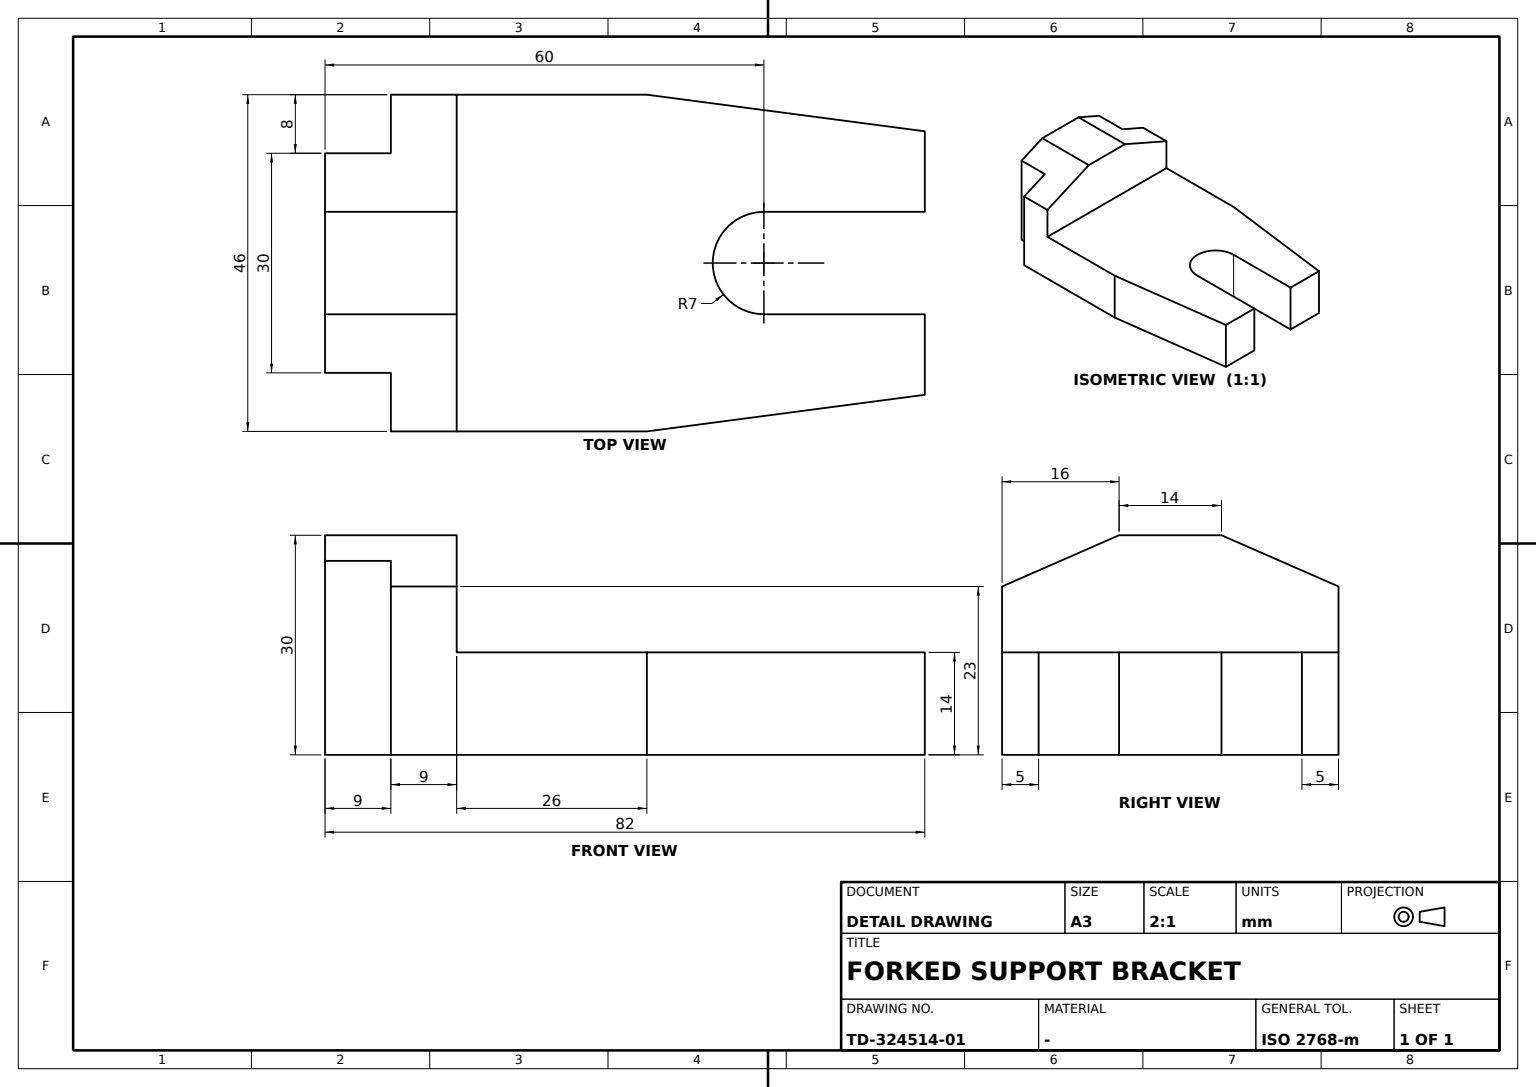
ISO-10303-21;
HEADER;
FILE_DESCRIPTION((''),'2;1');
FILE_NAME('','',(''),(''),'','','');
FILE_SCHEMA(('AUTOMOTIVE_DESIGN'));
ENDSEC;
DATA;
#1=APPLICATION_CONTEXT('');
#2=PRODUCT_CONTEXT('',#1,'mechanical');
#3=PRODUCT('','','',(#2));
#4=PRODUCT_DEFINITION_FORMATION('','',#3);
#5=PRODUCT_DEFINITION_CONTEXT('',#1,'design');
#6=PRODUCT_DEFINITION('','',#4,#5);
#7=PRODUCT_DEFINITION_SHAPE('','',#6);
#8=(LENGTH_UNIT()NAMED_UNIT(*)SI_UNIT(.MILLI.,.METRE.));
#9=(NAMED_UNIT(*)PLANE_ANGLE_UNIT()SI_UNIT($,.RADIAN.));
#10=(NAMED_UNIT(*)SI_UNIT($,.STERADIAN.)SOLID_ANGLE_UNIT());
#11=UNCERTAINTY_MEASURE_WITH_UNIT(LENGTH_MEASURE(0.005),#8,'distance_accuracy_value','');
#12=(GEOMETRIC_REPRESENTATION_CONTEXT(3)GLOBAL_UNCERTAINTY_ASSIGNED_CONTEXT((#11))GLOBAL_UNIT_ASSIGNED_CONTEXT((#8,#9,#10))REPRESENTATION_CONTEXT('',''));
#13=CARTESIAN_POINT('',(60.,-7.,14.));
#14=VERTEX_POINT('',#13);
#15=CARTESIAN_POINT('',(60.,-7.,0.));
#16=VERTEX_POINT('',#15);
#17=CARTESIAN_POINT('',(60.,-7.,-32.));
#18=DIRECTION('',(0.,0.,-1.));
#19=VECTOR('',#18,1000.);
#20=LINE('',#17,#19);
#21=EDGE_CURVE('',#14,#16,#20,.T.);
#22=ORIENTED_EDGE('',*,*,#21,.F.);
#23=CARTESIAN_POINT('',(82.,-7.,14.));
#24=VERTEX_POINT('',#23);
#25=DIRECTION('',(1.,0.,0.));
#26=VECTOR('',#25,1000.);
#27=LINE('',#13,#26);
#28=EDGE_CURVE('',#14,#24,#27,.T.);
#29=ORIENTED_EDGE('',*,*,#28,.T.);
#30=CARTESIAN_POINT('',(82.,-7.,0.));
#31=VERTEX_POINT('',#30);
#32=CARTESIAN_POINT('',(82.,-7.,-32.));
#33=DIRECTION('',(0.,0.,1.));
#34=VECTOR('',#33,1000.);
#35=LINE('',#32,#34);
#36=EDGE_CURVE('',#31,#24,#35,.T.);
#37=ORIENTED_EDGE('',*,*,#36,.F.);
#38=CARTESIAN_POINT('',(0.,-7.,0.));
#39=LINE('',#38,#26);
#40=EDGE_CURVE('',#16,#31,#39,.T.);
#41=ORIENTED_EDGE('',*,*,#40,.F.);
#42=EDGE_LOOP('',(#22,#29,#37,#41));
#43=FACE_BOUND('',#42,.T.);
#44=DIRECTION('',(0.,-1.,0.));
#45=AXIS2_PLACEMENT_3D('',#17,#44,#25);
#46=PLANE('',#45);
#47=ADVANCED_FACE('',(#43),#46,.F.);
#48=CARTESIAN_POINT('',(0.,-15.,0.));
#49=VERTEX_POINT('',#48);
#50=CARTESIAN_POINT('',(0.,-15.,26.5));
#51=VERTEX_POINT('',#50);
#52=CARTESIAN_POINT('',(0.,-15.,-16.));
#53=LINE('',#52,#34);
#54=EDGE_CURVE('',#49,#51,#53,.T.);
#55=ORIENTED_EDGE('',*,*,#54,.F.);
#56=CARTESIAN_POINT('',(9.,-15.,0.));
#57=VERTEX_POINT('',#56);
#58=DIRECTION('',(-1.,0.,0.));
#59=VECTOR('',#58,1000.);
#60=LINE('',#48,#59);
#61=EDGE_CURVE('',#57,#49,#60,.T.);
#62=ORIENTED_EDGE('',*,*,#61,.F.);
#63=CARTESIAN_POINT('',(9.,-15.,26.5));
#64=VERTEX_POINT('',#63);
#65=CARTESIAN_POINT('',(9.,-15.,-16.));
#66=LINE('',#65,#19);
#67=EDGE_CURVE('',#64,#57,#66,.T.);
#68=ORIENTED_EDGE('',*,*,#67,.F.);
#69=LINE('',#63,#59);
#70=EDGE_CURVE('',#64,#51,#69,.T.);
#71=ORIENTED_EDGE('',*,*,#70,.T.);
#72=EDGE_LOOP('',(#55,#62,#68,#71));
#73=FACE_BOUND('',#72,.T.);
#74=DIRECTION('',(0.,1.,0.));
#75=AXIS2_PLACEMENT_3D('',#65,#74,#33);
#76=PLANE('',#75);
#77=ADVANCED_FACE('',(#73),#76,.F.);
#78=CARTESIAN_POINT('',(44.,-23.,0.));
#79=VERTEX_POINT('',#78);
#80=CARTESIAN_POINT('',(44.,-23.,14.));
#81=VERTEX_POINT('',#80);
#82=CARTESIAN_POINT('',(44.,-23.,-32.));
#83=LINE('',#82,#34);
#84=EDGE_CURVE('',#79,#81,#83,.T.);
#85=ORIENTED_EDGE('',*,*,#84,.T.);
#86=CARTESIAN_POINT('',(18.,-23.,14.));
#87=VERTEX_POINT('',#86);
#88=CARTESIAN_POINT('',(82.,-23.,14.));
#89=LINE('',#88,#59);
#90=EDGE_CURVE('',#81,#87,#89,.T.);
#91=ORIENTED_EDGE('',*,*,#90,.T.);
#92=CARTESIAN_POINT('',(18.,-23.,23.));
#93=VERTEX_POINT('',#92);
#94=LINE('',#86,#34);
#95=EDGE_CURVE('',#87,#93,#94,.T.);
#96=ORIENTED_EDGE('',*,*,#95,.T.);
#97=CARTESIAN_POINT('',(9.,-23.,23.));
#98=VERTEX_POINT('',#97);
#99=CARTESIAN_POINT('',(-28.,-23.,23.));
#100=LINE('',#99,#26);
#101=EDGE_CURVE('',#98,#93,#100,.T.);
#102=ORIENTED_EDGE('',*,*,#101,.F.);
#103=CARTESIAN_POINT('',(9.,-23.,0.));
#104=VERTEX_POINT('',#103);
#105=CARTESIAN_POINT('',(9.,-23.,-16.));
#106=LINE('',#105,#34);
#107=EDGE_CURVE('',#104,#98,#106,.T.);
#108=ORIENTED_EDGE('',*,*,#107,.F.);
#109=CARTESIAN_POINT('',(0.,-23.,0.));
#110=LINE('',#109,#26);
#111=EDGE_CURVE('',#104,#79,#110,.T.);
#112=ORIENTED_EDGE('',*,*,#111,.T.);
#113=EDGE_LOOP('',(#85,#91,#96,#102,#108,#112));
#114=FACE_BOUND('',#113,.T.);
#115=AXIS2_PLACEMENT_3D('',#109,#44,#18);
#116=PLANE('',#115);
#117=ADVANCED_FACE('',(#114),#116,.T.);
#118=ORIENTED_EDGE('',*,*,#54,.T.);
#119=CARTESIAN_POINT('',(0.,-7.,30.));
#120=VERTEX_POINT('',#119);
#121=CARTESIAN_POINT('',(0.,-20.429508,24.12459));
#122=DIRECTION('',(0.,0.916157335,0.400818834));
#123=VECTOR('',#122,1000.);
#124=LINE('',#121,#123);
#125=EDGE_CURVE('',#51,#120,#124,.T.);
#126=ORIENTED_EDGE('',*,*,#125,.T.);
#127=CARTESIAN_POINT('',(0.,7.,30.));
#128=VERTEX_POINT('',#127);
#129=CARTESIAN_POINT('',(0.,-23.,30.));
#130=VECTOR('',#74,1000.);
#131=LINE('',#129,#130);
#132=EDGE_CURVE('',#120,#128,#131,.T.);
#133=ORIENTED_EDGE('',*,*,#132,.T.);
#134=CARTESIAN_POINT('',(0.,15.,26.5));
#135=VERTEX_POINT('',#134);
#136=CARTESIAN_POINT('',(0.,-18.180328,41.016393));
#137=DIRECTION('',(0.,0.916157335,-0.400818834));
#138=VECTOR('',#137,1000.);
#139=LINE('',#136,#138);
#140=EDGE_CURVE('',#128,#135,#139,.T.);
#141=ORIENTED_EDGE('',*,*,#140,.T.);
#142=CARTESIAN_POINT('',(0.,15.,0.));
#143=VERTEX_POINT('',#142);
#144=CARTESIAN_POINT('',(0.,15.,-16.));
#145=LINE('',#144,#34);
#146=EDGE_CURVE('',#143,#135,#145,.T.);
#147=ORIENTED_EDGE('',*,*,#146,.F.);
#148=LINE('',#109,#130);
#149=EDGE_CURVE('',#49,#143,#148,.T.);
#150=ORIENTED_EDGE('',*,*,#149,.F.);
#151=EDGE_LOOP('',(#118,#126,#133,#141,#147,#150));
#152=FACE_BOUND('',#151,.T.);
#153=AXIS2_PLACEMENT_3D('',#129,#25,#18);
#154=PLANE('',#153);
#155=ADVANCED_FACE('',(#152),#154,.F.);
#156=CARTESIAN_POINT('',(18.,23.,14.));
#157=VERTEX_POINT('',#156);
#158=CARTESIAN_POINT('',(18.,23.,23.));
#159=VERTEX_POINT('',#158);
#160=LINE('',#156,#34);
#161=EDGE_CURVE('',#157,#159,#160,.T.);
#162=ORIENTED_EDGE('',*,*,#161,.F.);
#163=CARTESIAN_POINT('',(44.,23.,14.));
#164=VERTEX_POINT('',#163);
#165=CARTESIAN_POINT('',(82.,23.,14.));
#166=LINE('',#165,#59);
#167=EDGE_CURVE('',#164,#157,#166,.T.);
#168=ORIENTED_EDGE('',*,*,#167,.F.);
#169=CARTESIAN_POINT('',(44.,23.,0.));
#170=VERTEX_POINT('',#169);
#171=CARTESIAN_POINT('',(44.,23.,-32.));
#172=LINE('',#171,#34);
#173=EDGE_CURVE('',#170,#164,#172,.T.);
#174=ORIENTED_EDGE('',*,*,#173,.F.);
#175=CARTESIAN_POINT('',(9.,23.,0.));
#176=VERTEX_POINT('',#175);
#177=CARTESIAN_POINT('',(0.,23.,0.));
#178=LINE('',#177,#26);
#179=EDGE_CURVE('',#176,#170,#178,.T.);
#180=ORIENTED_EDGE('',*,*,#179,.F.);
#181=CARTESIAN_POINT('',(9.,23.,23.));
#182=VERTEX_POINT('',#181);
#183=CARTESIAN_POINT('',(9.,23.,-16.));
#184=LINE('',#183,#34);
#185=EDGE_CURVE('',#176,#182,#184,.T.);
#186=ORIENTED_EDGE('',*,*,#185,.T.);
#187=CARTESIAN_POINT('',(-28.,23.,23.));
#188=LINE('',#187,#26);
#189=EDGE_CURVE('',#182,#159,#188,.T.);
#190=ORIENTED_EDGE('',*,*,#189,.T.);
#191=EDGE_LOOP('',(#162,#168,#174,#180,#186,#190));
#192=FACE_BOUND('',#191,.T.);
#193=AXIS2_PLACEMENT_3D('',#177,#44,#18);
#194=PLANE('',#193);
#195=ADVANCED_FACE('',(#192),#194,.F.);
#196=CARTESIAN_POINT('',(18.,7.,30.));
#197=VERTEX_POINT('',#196);
#198=LINE('',#196,#138);
#199=EDGE_CURVE('',#197,#159,#198,.T.);
#200=ORIENTED_EDGE('',*,*,#199,.T.);
#201=ORIENTED_EDGE('',*,*,#189,.F.);
#202=CARTESIAN_POINT('',(9.,15.,26.5));
#203=VERTEX_POINT('',#202);
#204=CARTESIAN_POINT('',(9.,30.606557,19.672131));
#205=LINE('',#204,#138);
#206=EDGE_CURVE('',#203,#182,#205,.T.);
#207=ORIENTED_EDGE('',*,*,#206,.F.);
#208=LINE('',#134,#26);
#209=EDGE_CURVE('',#135,#203,#208,.T.);
#210=ORIENTED_EDGE('',*,*,#209,.F.);
#211=ORIENTED_EDGE('',*,*,#140,.F.);
#212=CARTESIAN_POINT('',(-28.,7.,30.));
#213=LINE('',#212,#26);
#214=EDGE_CURVE('',#128,#197,#213,.T.);
#215=ORIENTED_EDGE('',*,*,#214,.T.);
#216=EDGE_LOOP('',(#200,#201,#207,#210,#211,#215));
#217=FACE_BOUND('',#216,.T.);
#218=DIRECTION('',(0.,-0.400818834,-0.916157335));
#219=AXIS2_PLACEMENT_3D('',#212,#218,#137);
#220=PLANE('',#219);
#221=ADVANCED_FACE('',(#217),#220,.F.);
#222=ORIENTED_EDGE('',*,*,#161,.T.);
#223=ORIENTED_EDGE('',*,*,#199,.F.);
#224=CARTESIAN_POINT('',(18.,-7.,30.));
#225=VERTEX_POINT('',#224);
#226=CARTESIAN_POINT('',(18.,-23.,30.));
#227=LINE('',#226,#130);
#228=EDGE_CURVE('',#225,#197,#227,.T.);
#229=ORIENTED_EDGE('',*,*,#228,.F.);
#230=LINE('',#92,#123);
#231=EDGE_CURVE('',#93,#225,#230,.T.);
#232=ORIENTED_EDGE('',*,*,#231,.F.);
#233=ORIENTED_EDGE('',*,*,#95,.F.);
#234=LINE('',#86,#130);
#235=EDGE_CURVE('',#87,#157,#234,.T.);
#236=ORIENTED_EDGE('',*,*,#235,.T.);
#237=EDGE_LOOP('',(#222,#223,#229,#232,#233,#236));
#238=FACE_BOUND('',#237,.T.);
#239=AXIS2_PLACEMENT_3D('',#86,#58,#33);
#240=PLANE('',#239);
#241=ADVANCED_FACE('',(#238),#240,.F.);
#242=ORIENTED_EDGE('',*,*,#21,.T.);
#243=CARTESIAN_POINT('',(60.,7.,0.));
#244=VERTEX_POINT('',#243);
#245=CARTESIAN_POINT('',(60.,0.,0.));
#246=AXIS2_PLACEMENT_3D('',#245,#33,#25);
#247=CIRCLE('',#246,7.);
#248=EDGE_CURVE('',#244,#16,#247,.T.);
#249=ORIENTED_EDGE('',*,*,#248,.F.);
#250=CARTESIAN_POINT('',(60.,7.,14.));
#251=VERTEX_POINT('',#250);
#252=CARTESIAN_POINT('',(60.,7.,-32.));
#253=LINE('',#252,#19);
#254=EDGE_CURVE('',#251,#244,#253,.T.);
#255=ORIENTED_EDGE('',*,*,#254,.F.);
#256=CARTESIAN_POINT('',(60.,0.,14.));
#257=AXIS2_PLACEMENT_3D('',#256,#33,#74);
#258=CIRCLE('',#257,7.);
#259=EDGE_CURVE('',#251,#14,#258,.T.);
#260=ORIENTED_EDGE('',*,*,#259,.T.);
#261=EDGE_LOOP('',(#242,#249,#255,#260));
#262=FACE_BOUND('',#261,.T.);
#263=CARTESIAN_POINT('',(60.,0.,-32.));
#264=AXIS2_PLACEMENT_3D('',#263,#33,#25);
#265=CYLINDRICAL_SURFACE('',#264,7.);
#266=ADVANCED_FACE('',(#262),#265,.F.);
#267=LINE('',#103,#130);
#268=EDGE_CURVE('',#104,#57,#267,.T.);
#269=ORIENTED_EDGE('',*,*,#268,.F.);
#270=ORIENTED_EDGE('',*,*,#107,.T.);
#271=CARTESIAN_POINT('',(9.,-37.321311,16.734426));
#272=LINE('',#271,#123);
#273=EDGE_CURVE('',#98,#64,#272,.T.);
#274=ORIENTED_EDGE('',*,*,#273,.T.);
#275=ORIENTED_EDGE('',*,*,#67,.T.);
#276=EDGE_LOOP('',(#269,#270,#274,#275));
#277=FACE_BOUND('',#276,.T.);
#278=AXIS2_PLACEMENT_3D('',#105,#25,#18);
#279=PLANE('',#278);
#280=ADVANCED_FACE('',(#277),#279,.F.);
#281=CARTESIAN_POINT('',(9.,15.,0.));
#282=VERTEX_POINT('',#281);
#283=CARTESIAN_POINT('',(9.,15.,-16.));
#284=LINE('',#283,#19);
#285=EDGE_CURVE('',#203,#282,#284,.T.);
#286=ORIENTED_EDGE('',*,*,#285,.T.);
#287=LINE('',#142,#26);
#288=EDGE_CURVE('',#143,#282,#287,.T.);
#289=ORIENTED_EDGE('',*,*,#288,.F.);
#290=ORIENTED_EDGE('',*,*,#146,.T.);
#291=ORIENTED_EDGE('',*,*,#209,.T.);
#292=EDGE_LOOP('',(#286,#289,#290,#291));
#293=FACE_BOUND('',#292,.T.);
#294=AXIS2_PLACEMENT_3D('',#144,#44,#18);
#295=PLANE('',#294);
#296=ADVANCED_FACE('',(#293),#295,.F.);
#297=CARTESIAN_POINT('',(82.,7.,14.));
#298=VERTEX_POINT('',#297);
#299=LINE('',#297,#59);
#300=EDGE_CURVE('',#298,#251,#299,.T.);
#301=ORIENTED_EDGE('',*,*,#300,.T.);
#302=ORIENTED_EDGE('',*,*,#254,.T.);
#303=CARTESIAN_POINT('',(82.,7.,0.));
#304=VERTEX_POINT('',#303);
#305=CARTESIAN_POINT('',(0.,7.,0.));
#306=LINE('',#305,#59);
#307=EDGE_CURVE('',#304,#244,#306,.T.);
#308=ORIENTED_EDGE('',*,*,#307,.F.);
#309=CARTESIAN_POINT('',(82.,7.,-32.));
#310=LINE('',#309,#34);
#311=EDGE_CURVE('',#304,#298,#310,.T.);
#312=ORIENTED_EDGE('',*,*,#311,.T.);
#313=EDGE_LOOP('',(#301,#302,#308,#312));
#314=FACE_BOUND('',#313,.T.);
#315=AXIS2_PLACEMENT_3D('',#309,#74,#58);
#316=PLANE('',#315);
#317=ADVANCED_FACE('',(#314),#316,.F.);
#318=CARTESIAN_POINT('',(82.,-18.,0.));
#319=VERTEX_POINT('',#318);
#320=CARTESIAN_POINT('',(0.748809,-28.690946,0.));
#321=DIRECTION('',(-0.991454296,-0.130454513,0.));
#322=VECTOR('',#321,1000.);
#323=LINE('',#320,#322);
#324=EDGE_CURVE('',#319,#79,#323,.T.);
#325=ORIENTED_EDGE('',*,*,#324,.F.);
#326=CARTESIAN_POINT('',(82.,-18.,14.));
#327=VERTEX_POINT('',#326);
#328=CARTESIAN_POINT('',(82.,-18.,-32.));
#329=LINE('',#328,#34);
#330=EDGE_CURVE('',#319,#327,#329,.T.);
#331=ORIENTED_EDGE('',*,*,#330,.T.);
#332=LINE('',#326,#322);
#333=EDGE_CURVE('',#327,#81,#332,.T.);
#334=ORIENTED_EDGE('',*,*,#333,.T.);
#335=ORIENTED_EDGE('',*,*,#84,.F.);
#336=EDGE_LOOP('',(#325,#331,#334,#335));
#337=FACE_BOUND('',#336,.T.);
#338=DIRECTION('',(-0.130454513,0.991454296,0.));
#339=AXIS2_PLACEMENT_3D('',#328,#338,#321);
#340=PLANE('',#339);
#341=ADVANCED_FACE('',(#337),#340,.F.);
#342=ORIENTED_EDGE('',*,*,#167,.T.);
#343=ORIENTED_EDGE('',*,*,#235,.F.);
#344=ORIENTED_EDGE('',*,*,#90,.F.);
#345=ORIENTED_EDGE('',*,*,#333,.F.);
#346=LINE('',#88,#130);
#347=EDGE_CURVE('',#327,#24,#346,.T.);
#348=ORIENTED_EDGE('',*,*,#347,.T.);
#349=ORIENTED_EDGE('',*,*,#28,.F.);
#350=ORIENTED_EDGE('',*,*,#259,.F.);
#351=ORIENTED_EDGE('',*,*,#300,.F.);
#352=CARTESIAN_POINT('',(82.,18.,14.));
#353=VERTEX_POINT('',#352);
#354=EDGE_CURVE('',#298,#353,#346,.T.);
#355=ORIENTED_EDGE('',*,*,#354,.T.);
#356=DIRECTION('',(0.991454296,-0.130454513,0.));
#357=VECTOR('',#356,1000.);
#358=LINE('',#163,#357);
#359=EDGE_CURVE('',#164,#353,#358,.T.);
#360=ORIENTED_EDGE('',*,*,#359,.F.);
#361=EDGE_LOOP('',(#342,#343,#344,#345,#348,#349,#350,#351,#355,#360));
#362=FACE_BOUND('',#361,.T.);
#363=AXIS2_PLACEMENT_3D('',#88,#18,#58);
#364=PLANE('',#363);
#365=ADVANCED_FACE('',(#362),#364,.F.);
#366=ORIENTED_EDGE('',*,*,#228,.T.);
#367=ORIENTED_EDGE('',*,*,#214,.F.);
#368=ORIENTED_EDGE('',*,*,#132,.F.);
#369=CARTESIAN_POINT('',(-28.,-7.,30.));
#370=LINE('',#369,#26);
#371=EDGE_CURVE('',#120,#225,#370,.T.);
#372=ORIENTED_EDGE('',*,*,#371,.T.);
#373=EDGE_LOOP('',(#366,#367,#368,#372));
#374=FACE_BOUND('',#373,.T.);
#375=AXIS2_PLACEMENT_3D('',#226,#18,#58);
#376=PLANE('',#375);
#377=ADVANCED_FACE('',(#374),#376,.F.);
#378=ORIENTED_EDGE('',*,*,#173,.T.);
#379=ORIENTED_EDGE('',*,*,#359,.T.);
#380=CARTESIAN_POINT('',(82.,18.,0.));
#381=VERTEX_POINT('',#380);
#382=CARTESIAN_POINT('',(82.,18.,-32.));
#383=LINE('',#382,#34);
#384=EDGE_CURVE('',#381,#353,#383,.T.);
#385=ORIENTED_EDGE('',*,*,#384,.F.);
#386=CARTESIAN_POINT('',(6.698434,27.908101,0.));
#387=LINE('',#386,#357);
#388=EDGE_CURVE('',#170,#381,#387,.T.);
#389=ORIENTED_EDGE('',*,*,#388,.F.);
#390=EDGE_LOOP('',(#378,#379,#385,#389));
#391=FACE_BOUND('',#390,.T.);
#392=DIRECTION('',(-0.130454513,-0.991454296,0.));
#393=AXIS2_PLACEMENT_3D('',#171,#392,#356);
#394=PLANE('',#393);
#395=ADVANCED_FACE('',(#391),#394,.F.);
#396=ORIENTED_EDGE('',*,*,#354,.F.);
#397=ORIENTED_EDGE('',*,*,#311,.F.);
#398=CARTESIAN_POINT('',(82.,-23.,0.));
#399=LINE('',#398,#130);
#400=EDGE_CURVE('',#304,#381,#399,.T.);
#401=ORIENTED_EDGE('',*,*,#400,.T.);
#402=ORIENTED_EDGE('',*,*,#384,.T.);
#403=EDGE_LOOP('',(#396,#397,#401,#402));
#404=FACE_BOUND('',#403,.T.);
#405=AXIS2_PLACEMENT_3D('',#398,#58,#33);
#406=PLANE('',#405);
#407=ADVANCED_FACE('',(#404),#406,.F.);
#408=ORIENTED_EDGE('',*,*,#61,.T.);
#409=ORIENTED_EDGE('',*,*,#149,.T.);
#410=ORIENTED_EDGE('',*,*,#288,.T.);
#411=EDGE_CURVE('',#282,#176,#267,.T.);
#412=ORIENTED_EDGE('',*,*,#411,.T.);
#413=ORIENTED_EDGE('',*,*,#179,.T.);
#414=ORIENTED_EDGE('',*,*,#388,.T.);
#415=ORIENTED_EDGE('',*,*,#400,.F.);
#416=ORIENTED_EDGE('',*,*,#307,.T.);
#417=ORIENTED_EDGE('',*,*,#248,.T.);
#418=ORIENTED_EDGE('',*,*,#40,.T.);
#419=EDGE_CURVE('',#319,#31,#399,.T.);
#420=ORIENTED_EDGE('',*,*,#419,.F.);
#421=ORIENTED_EDGE('',*,*,#324,.T.);
#422=ORIENTED_EDGE('',*,*,#111,.F.);
#423=ORIENTED_EDGE('',*,*,#268,.T.);
#424=EDGE_LOOP('',(#408,#409,#410,#412,#413,#414,#415,#416,#417,#418,#420,#421,#422,#423));
#425=FACE_BOUND('',#424,.T.);
#426=AXIS2_PLACEMENT_3D('',#109,#33,#25);
#427=PLANE('',#426);
#428=ADVANCED_FACE('',(#425),#427,.F.);
#429=ORIENTED_EDGE('',*,*,#419,.T.);
#430=ORIENTED_EDGE('',*,*,#36,.T.);
#431=ORIENTED_EDGE('',*,*,#347,.F.);
#432=ORIENTED_EDGE('',*,*,#330,.F.);
#433=EDGE_LOOP('',(#429,#430,#431,#432));
#434=FACE_BOUND('',#433,.T.);
#435=ADVANCED_FACE('',(#434),#406,.F.);
#436=ORIENTED_EDGE('',*,*,#411,.F.);
#437=ORIENTED_EDGE('',*,*,#285,.F.);
#438=ORIENTED_EDGE('',*,*,#206,.T.);
#439=ORIENTED_EDGE('',*,*,#185,.F.);
#440=EDGE_LOOP('',(#436,#437,#438,#439));
#441=FACE_BOUND('',#440,.T.);
#442=AXIS2_PLACEMENT_3D('',#283,#25,#74);
#443=PLANE('',#442);
#444=ADVANCED_FACE('',(#441),#443,.F.);
#445=ORIENTED_EDGE('',*,*,#125,.F.);
#446=ORIENTED_EDGE('',*,*,#70,.F.);
#447=ORIENTED_EDGE('',*,*,#273,.F.);
#448=ORIENTED_EDGE('',*,*,#101,.T.);
#449=ORIENTED_EDGE('',*,*,#231,.T.);
#450=ORIENTED_EDGE('',*,*,#371,.F.);
#451=EDGE_LOOP('',(#445,#446,#447,#448,#449,#450));
#452=FACE_BOUND('',#451,.T.);
#453=DIRECTION('',(0.,0.400818834,-0.916157335));
#454=AXIS2_PLACEMENT_3D('',#99,#453,#122);
#455=PLANE('',#454);
#456=ADVANCED_FACE('',(#452),#455,.F.);
#457=CLOSED_SHELL('',(#47,#77,#117,#155,#195,#221,#241,#266,#280,#296,#317,#341,#365,#377,#395,#407,#428,#435,#444,#456));
#458=MANIFOLD_SOLID_BREP('',#457);
#459=ADVANCED_BREP_SHAPE_REPRESENTATION('',(#458),#12);
#460=SHAPE_DEFINITION_REPRESENTATION(#7,#459);
ENDSEC;
END-ISO-10303-21;
